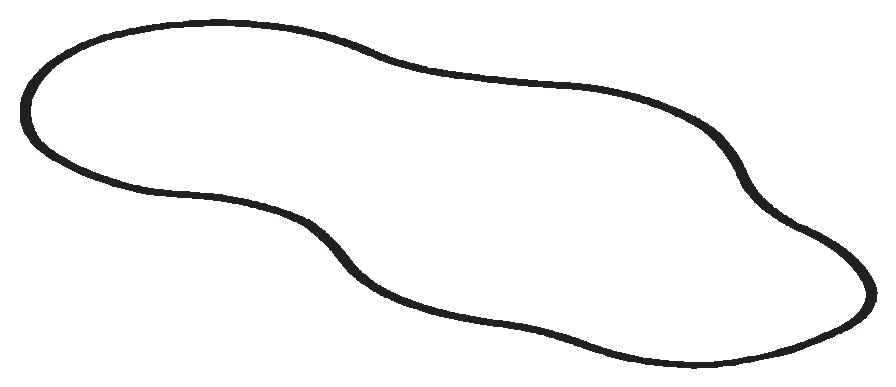
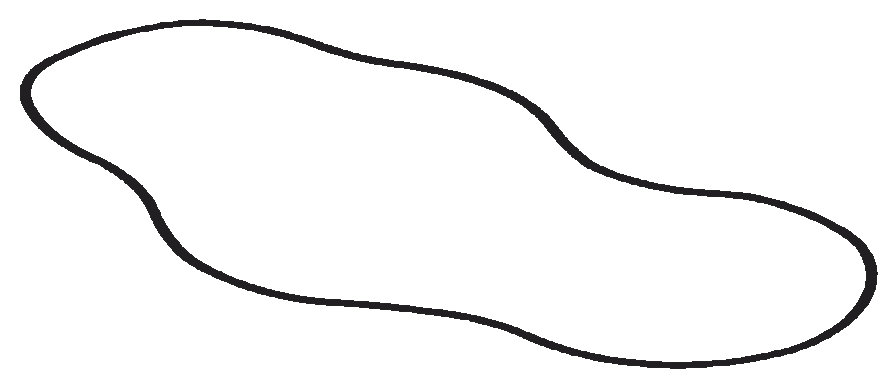
# SketchUp Ruby script. Lengths in inches.
U = 1.inch
M = Sketchup.active_model
def pt(a) = Geom::Point3d.new(a.map { |v| v * U })
def face(e, loops, mat)
  f = e.add_face(loops[0].map { |a| pt(a) })
  loops[1..].each { |l| e.add_face(l.map { |a| pt(a) }).erase! }
  f.material = f.back_material = mat if mat
  f
end
# faces: each face lists its corners as indices into pts; further lists are holes
def faces(e, pts, list, mat = nil) = list.each { |f| face(e, (f[0].is_a?(Array) ? f : [f]).map { |l| l.map { |i| pts[i] } }, mat) }
# xy, xz, yz: faces in a plane at the given z, y or x. An outline is a flat list of corners, or four numbers for a rectangle; further outlines are holes
def ring(l) = l.size == 4 ? [[l[0], l[1]], [l[2], l[1]], [l[2], l[3]], [l[0], l[3]]] : l.each_slice(2).to_a
def flat(e, list, mat, &to3) = list.each { |f| face(e, (f[0].is_a?(Array) ? f : [f]).map { |l| ring(l).map { |u, v| to3.(u, v) } }, mat) }
def xy(e, z, list, mat = nil) = flat(e, list, mat) { |x, y| [x, y, z] }
def xz(e, y, list, mat = nil) = flat(e, list, mat) { |x, z| [x, y, z] }
def yz(e, x, list, mat = nil) = flat(e, list, mat) { |y, z| [x, y, z] }
def lines(e, pts, list) = list.each { |a, b| e.add_line(pt(pts[a]), pt(pts[b])) }
# prism: a flat outline (further loops are holes) pulled along v
def prism(e, loops, v, mat = nil)
  f = face(e, loops, mat); d = Geom::Vector3d.new(v.map { |x| x * U })
  f.pushpull(f.normal.samedirection?(d) ? d.length : -d.length)
end
def box(e, o, s, mat = nil) = prism(e, [[o, [o[0] + s[0], o[1], o[2]], [o[0] + s[0], o[1] + s[1], o[2]], [o[0], o[1] + s[1], o[2]]]], [0, 0, s[2]], mat)
def at(x, y, z, deg = 0) = Geom::Transformation.translation(pt([x, y, z])) * Geom::Transformation.rotation(ORIGIN, Z_AXIS, deg.degrees)
def axes(o, x, y, z) = Geom::Transformation.new([*x, 0, *y, 0, *z, 0, *pt(o).to_a, 1])
def part(name) = M.definitions.add(name)
# library, detail: a bought-in or finely detailed component or shape, given as its bounding box
def library(name, o, s) = part(name).tap { |d| box(d.entities, o, s) }
def detail(e, o, s) = box(e.add_group.entities, o, s)
def put(e, d, t, mat = nil) = e.add_instance(d, t).tap { |i| i.material = mat if mat }
def group(e, t, mat = nil) = e.add_group.tap { |g| g.transformation = t; g.material = mat if mat }.entities
root = M.entities
M.materials.add("Marble_07_1K").color = [36, 34, 36]
xy(root,19,[[[347.23,772.58,347.79,772.58,348.02,772.59,348.13,772.6,348.24,772.6,348.79,772.65,348.99,772.67,349.09,772.69,349.18,772.7,349.28,772.71,349.36,772.72,349.45,772.74,349.61,772.76,349.6875,772.78,349.77,772.79,349.85,772.8,349.93,772.82,350,772.83,350.08,772.85,350.16,772.86,350.32,772.9,350.4,772.91,350.47,772.93,350.55,772.95,350.63,772.96,350.71,772.98,350.78,773,350.86,773.02,350.9375,773.04,351.02,773.06,351.09,773.08,351.33,773.14,351.4,773.16,351.56,773.2,351.63,773.23,351.79,773.27,351.86,773.29,351.9375,773.32,352.01,773.34,352.09,773.37,352.17,773.39,352.24,773.42,352.32,773.44,352.39,773.47,352.47,773.49,352.54,773.52,352.62,773.54,352.69,773.57,352.77,773.6,352.84,773.625,352.92,773.65,352.99,773.68,353.07,773.71,353.14,773.74,353.22,773.77,353.36,773.83,353.4375,773.86,353.51,773.89,353.65,773.95,353.73,773.98,353.8,774.01,353.875,774.04,353.95,774.08,354.11,774.14,354.19,774.18,354.35,774.24,354.4375,774.28,354.52,774.3125,354.61,774.35,354.69,774.38,354.78,774.41,354.86,774.44,354.95,774.47,355.03,774.51,355.12,774.54,355.2,774.5625,355.29,774.59,355.46,774.65,355.55,774.68,355.63,774.7,355.72,774.73,355.81,774.75,355.89,774.78,356.07,774.82,356.16,774.85,356.24,774.87,356.6,774.95,356.68,774.97,356.77,774.98,357.04,775.04,357.125,775.05,357.22,775.07,357.3,775.08,357.39,775.09,357.48,775.11,358.11,775.18,358.2,775.1875,358.29,775.2,358.38,775.2,358.47,775.21,358.5625,775.21,358.65,775.22,358.74,775.22,358.84,775.23,359.12,775.23,359.22,775.24,359.46,775.24,359.6,775.25,359.76,775.25,359.9375,775.26,360.14,775.27,360.36,775.29,360.6,775.31,360.85,775.33,361.39,775.39,361.67,775.43,361.96,775.48,362.24,775.53,362.52,775.59,362.8,775.66,363.08,775.74,363.35,775.82,363.625,775.91,363.9,776.01,364.17,776.11,364.4375,776.22,364.7,776.34,364.96,776.46,365.22,776.59,365.48,776.73,365.98,777.02,366.22,777.18,366.7,777.52,366.9375,777.7,367.17,777.9,367.41,778.11,367.64,778.35,367.875,778.6,368.11,778.875,368.35,779.18,368.59,779.52,368.85,779.9,369.11,780.34,369.4,780.85,369.7,781.4375,370.02,782.11,370.37,782.88,370.59,783.7,370.76,784.42,370.9,785.05,371.01,785.59,371.09,786.06,371.15,786.45,371.19,786.79,371.22,787.07,371.25,787.3,371.26,787.49,371.28,787.65,371.29,787.78,371.29,788.17,371.28,788.23,371.28,788.36,371.27,788.43,371.27,788.49,371.26,788.56,371.25,788.62,371.24,788.6875,371.24,788.75,371.23,788.81,371.22,788.88,371.21,788.94,371.2,789.01,371.18,789.07,371.17,789.13,371.16,789.2,371.14,789.26,371.13,789.32,371.12,789.39,371.08,789.51,371.07,789.58,371.01,789.76,370.99,789.83,370.89,790.13,370.86,790.19,370.84,790.25,370.8125,790.3125,370.79,790.375,370.76,790.43,370.74,790.49,370.65,790.67,370.625,790.73,370.51,790.96,370.47,791.01,370.44,791.07,370.41,791.125,370.375,791.18,370.34,791.24,370.31,791.29,370.27,791.35,370.24,791.4,370.2,791.46,370.16,791.51,370.125,791.5625,370.09,791.61,370.05,791.67,369.73,792.07,369.68,792.12,369.64,792.17,369.55,792.26,369.51,792.3125,369.46,792.36,369.41,792.4,369.37,792.45,369.32,792.49,369.23,792.58,369.13,792.67,369.03,792.75,368.99,792.79,368.9375,792.83,368.89,792.87,368.84,792.91,368.8,792.94,368.7,793.02,368.66,793.05,368.61,793.09,368.53,793.15,368.5,793.18,368.46,793.2,368.43,793.22,368.41,793.24,368.38,793.26,368.35,793.29,368.33,793.3,368.32,793.31,368.3,793.32,368.28,793.34,368.27,793.34,368.25,793.35,368.24,793.37,368.22,793.38,368.16,793.42,368.125,793.44,368.08,793.47,367.98,793.55,367.92,793.59,367.78,793.67,367.71,793.72,367.64,793.76,367.57,793.81,367.5,793.85,367.43,793.9,367.36,793.9375,367.28,793.98,367.21,794.03,367.07,794.11,366.99,794.15,366.85,794.23,366.77,794.27,366.7,794.31,366.62,794.35,366.55,794.39,366.47,794.43,366.4,794.46,366.32,794.5,366.25,794.54,366.17,794.57,366.09,794.61,366.02,794.64,365.94,794.68,365.86,794.71,365.79,794.74,365.71,794.78,365.55,794.84,365.48,794.875,365.4,794.9,364.84,795.11,364.76,795.13,364.68,795.16,364.6,795.1875,364.52,795.21,364.44,795.24,364.36,795.26,364.28,795.29,364.04,795.35,363.88,795.4,363.8,795.42,363.71,795.4375,363.63,795.46,363.39,795.52,363.3,795.53,363.14,795.57,363.06,795.58,362.97,795.6,362.89,795.61,362.81,795.63,362.73,795.64,362.64,795.66,362.48,795.68,362.39,795.69,362.3125,795.7,362.23,795.71,362.15,795.73,362.0625,795.73,361.98,795.74,361.9,795.75,361.81,795.76,361.65,795.78,361.56,795.78,361.47,795.79,361.17,795.82,360.95,795.84,360.83,795.85,360.71,795.87,360.47,795.89,359.99,795.97,359.76,796.01,359.64,796.03,359.52,796.06,359.4,796.08,359.28,796.11,359.17,796.14,359.05,796.16,358.93,796.19,358.82,796.23,358.7,796.26,358.59,796.29,358.47,796.33,358.36,796.36,358.24,796.4,358.13,796.4375,358.01,796.48,357.9,796.52,357.79,796.5625,357.68,796.6,357.5625,796.65,357.45,796.69,357.01,796.89,356.9,796.9375,356.79,796.99,356.68,797.04,356.58,797.1,356.47,797.15,356.36,797.21,356.26,797.27,356.15,797.32,356.05,797.38,355.94,797.44,355.84,797.51,355.64,797.63,355.53,797.7,355.43,797.76,355.13,797.97,355.04,798.04,354.9375,798.11,354.84,798.18,354.74,798.25,354.65,798.33,354.55,798.4,354.46,798.47,354.29,798.61,354.02,798.82,353.93,798.9,353.71,799.08,353.57,799.19,353.42,799.3,353.27,799.42,353.14,799.52,353.02,799.61,352.91,799.6875,352.81,799.75,352.73,799.8125,352.65,799.87,352.51,799.97,352.45,800.01,352.38,800.05,352.32,800.1,352.26,800.14,352.21,800.18,352.15,800.21,352.09,800.25,352.04,800.29,351.98,800.33,351.92,800.36,351.86,800.4,351.81,800.4375,351.75,800.47,351.69,800.51,351.63,800.54,351.58,800.58,351.52,800.62,351.46,800.65,351.4,800.6875,351.34,800.72,351.29,800.76,351.23,800.79,351.17,800.83,351.11,800.86,351.05,800.9,350.93,800.96,350.875,801,350.82,801.03,350.76,801.06,350.7,801.1,350.58,801.16,350.52,801.2,350.46,801.23,350.41,801.26,350.35,801.29,350.3,801.3125,350.25,801.34,350.21,801.36,350.16,801.39,350.08,801.43,350.05,801.45,350.01,801.46,349.97,801.48,349.94,801.5,349.91,801.51,349.83,801.55,349.8,801.56,349.76,801.58,349.73,801.6,349.69,801.61,349.66,801.63,349.62,801.64,349.59,801.66,349.55,801.68,349.51,801.69,349.47,801.71,349.43,801.72,349.35,801.76,349.2,801.82,349.13,801.84,349.0625,801.87,348.98,801.9,348.89,801.93,348.79,801.97,348.68,802,348.59,802.03,348.51,802.05,348.4375,802.07,348.375,802.09,348.32,802.11,348.26,802.12,348.22,802.13,348.17,802.14,348.125,802.16,348.08,802.17,348,802.19,347.97,802.19,347.85,802.22,347.8125,802.23,347.78,802.24,347.74,802.24,347.62,802.27,347.58,802.27,347.55,802.28,347.47,802.3,347.43,802.3,347.39,802.31,347.35,802.3125,347.28,802.33,347.24,802.33,347.2,802.34,347.16,802.34,347.125,802.35,347.09,802.35,347.05,802.36,347.01,802.36,346.97,802.37,346.89,802.38,346.85,802.38,346.8,802.39,346.74,802.39,346.67,802.4,346.59,802.41,346.49,802.42,346.38,802.43,346.25,802.4375,346.1,802.45,345.9375,802.46,345.76,802.47,345.56,802.48,345.34,802.49,345.11,802.5,344.85,802.51,344.58,802.52,344.29,802.52,343.99,802.51,343.67,802.5,343.34,802.47,342.99,802.4375,342.63,802.39,342.3,802.32,342.01,802.26,341.76,802.2,341.55,802.15,341.36,802.11,341.21,802.07,341.07,802.03,340.96,802,340.87,801.97,340.79,801.95,340.72,801.93,340.66,801.92,340.61,801.9,340.57,801.89,340.54,801.88,340.5,801.87,340.47,801.86,340.44,801.84,340.4,801.83,340.37,801.82,340.33,801.81,340.27,801.79,340.23,801.77,340.17,801.75,340.13,801.74,340.1,801.73,340.07,801.71,340.03,801.7,339.97,801.68,339.94,801.66,339.9,801.65,339.87,801.64,339.84,801.625,339.8,801.61,339.74,801.59,339.71,801.57,339.67,801.56,339.64,801.54,339.61,801.53,339.57,801.52,339.54,801.5,339.48,801.48,339.44,801.46,339.41,801.45,339.38,801.43,339.35,801.42,339.3125,801.4,339.28,801.39,339.24,801.37,339.21,801.35,339.17,801.33,339.125,801.3125,339.08,801.29,339.03,801.27,338.98,801.24,338.92,801.21,338.85,801.17,338.77,801.13,338.68,801.09,338.59,801.04,338.45,800.96,338.39,800.92,338.34,800.89,338.29,800.87,338.25,800.84,338.17,800.8,338.14,800.77,338.11,800.75,338.07,800.73,338.04,800.71,338.01,800.7,337.95,800.66,337.93,800.64,337.89,800.62,337.86,800.6,337.78,800.54,337.72,800.51,337.65,800.47,337.57,800.42,337.48,800.37,337.375,800.3,337.26,800.23,337.13,800.16,337,800.08,336.86,800,336.71,799.91,336.57,799.83,336.42,799.75,336.27,799.66,335.97,799.5,335.83,799.42,335.53,799.26,335.375,799.18,335.23,799.1,335.08,799.02,334.92,798.95,334.77,798.87,334.62,798.8,334.47,798.72,334.31,798.65,334.16,798.57,334.01,798.5,333.85,798.43,333.55,798.29,333.41,798.22,333.27,798.16,333.14,798.1,333.02,798.04,332.91,797.99,332.81,797.94,332.71,797.9,332.625,797.85,332.54,797.8125,332.46,797.77,332.38,797.74,332.31,797.7,332.23,797.67,332.15,797.63,332.08,797.6,332,797.57,331.93,797.54,331.85,797.5,331.78,797.47,331.62,797.41,331.55,797.38,331.39,797.32,331.32,797.29,331.24,797.27,331.08,797.21,331.01,797.1875,330.93,797.16,330.85,797.13,330.77,797.11,330.69,797.08,330.62,797.06,330.54,797.04,330.46,797.01,330.14,796.93,330.0625,796.91,329.98,796.89,329.5,796.77,329.41,796.76,329.23,796.72,329.13,796.7,329.02,796.68,328.91,796.67,328.79,796.65,328.65,796.625,328.49,796.6,328.3125,796.58,328.11,796.56,327.88,796.53,327.65,796.52,327.45,796.51,327.27,796.5,327.11,796.5,326.97,796.49,326.62,796.49,326.52,796.5,326.25,796.5,326.16,796.51,326.07,796.51,325.99,796.52,325.9,796.52,325.82,796.53,325.73,796.53,325.64,796.54,325.54,796.55,325.4375,796.55,325.33,796.56,324.78,796.56,324.62,796.55,324.45,796.55,324.28,796.54,324.1,796.53,323.92,796.51,323.73,796.5,323.37,796.46,323.18,796.4375,323,796.41,322.82,796.39,322.64,796.36,322.46,796.32,322.28,796.29,321.74,796.17,321.5625,796.125,321.39,796.08,321.03,795.98,320.86,795.93,320.68,795.87,320.51,795.8125,320.34,795.75,320.16,795.69,319.82,795.56,319.48,795.42,319.32,795.34,319.15,795.27,318.98,795.1875,318.82,795.11,318.65,795.03,317.85,794.58,317.7,794.48,317.54,794.39,317.39,794.29,317.23,794.1875,317.08,794.08,316.93,793.98,316.78,793.87,316.64,793.76,316.49,793.65,316.35,793.54,316.2,793.42,316.0625,793.3,315.92,793.19,315.79,793.0625,315.65,792.94,315.51,792.82,315.38,792.69,315.25,792.5625,315.12,792.43,314.99,792.3,314.87,792.17,314.74,792.04,314.26,791.48,314.15,791.34,314.03,791.19,313.92,791.05,313.8125,790.9,313.7,790.75,313.6,790.6,313.49,790.45,313.39,790.29,313.28,790.13,313.17,789.96,313.0625,789.78,312.95,789.59,312.83,789.39,312.72,789.19,312.48,788.77,312.26,788.35,312.16,788.14,312.07,787.94,311.99,787.75,311.92,787.57,311.86,787.39,311.8,787.22,311.75,787.05,311.63,786.57,311.6,786.41,311.56,786.25,311.54,786.09,311.51,785.9375,311.48,785.78,311.42,785.3,311.41,785.15,311.39,784.99,311.38,784.84,311.37,784.6875,311.36,784.54,311.36,784.4,311.35,784.27,311.35,783.81,311.36,783.71,311.36,783.53,311.37,783.45,311.37,783.36,311.38,783.28,311.38,783.2,311.39,783.12,311.39,783.03,311.4,782.9375,311.41,782.84,311.42,782.74,311.4375,782.625,311.46,782.5,311.48,782.37,311.52,782.09,311.55,781.9375,311.58,781.79,311.61,781.63,311.65,781.47,311.68,781.32,311.72,781.16,311.76,781.01,311.81,780.85,311.85,780.7,311.9,780.55,311.95,780.39,312.05,780.09,312.29,779.49,312.35,779.35,312.49,779.05,312.63,778.77,312.7,778.62,312.78,778.47,312.96,778.17,313.06,778.01,313.16,777.84,313.27,777.67,313.4,777.48,313.54,777.28,313.7,777.0625,313.89,776.82,314.11,776.54,314.36,776.24,314.66,775.89,314.99,775.59,315.3,775.33,315.57,775.1,315.81,774.9,316.03,774.74,316.24,774.59,316.43,774.46,316.61,774.34,316.78,774.24,316.96,774.14,317.13,774.04,317.32,773.96,317.51,773.87,317.71,773.79,317.92,773.71,318.16,773.63,318.41,773.55,318.68,773.47,318.97,773.4,319.28,773.32,319.59,773.25,319.91,773.1875,320.24,773.13,320.58,773.08,320.91,773.04,321.25,773,321.58,772.98,321.92,772.96,322.59,772.96,322.93,772.97,323.27,772.99,323.93,773.05,324.26,773.09,324.57,773.14,324.87,773.1875,325.15,773.24,325.42,773.29,325.65,773.35,325.87,773.4,326.23,773.5,326.39,773.55,326.54,773.61,326.68,773.67,326.83,773.74,326.99,773.8125,327.15,773.9,327.32,773.99,327.5,774.08,327.68,774.18,327.87,774.28,328.05,774.39,328.24,774.49,328.42,774.6,328.6,774.7,328.77,774.8,328.9375,774.89,329.1,774.99,329.27,775.08,329.43,775.17,329.59,775.25,329.75,775.34,329.92,775.42,330.08,775.49,330.24,775.57,330.4,775.64,330.74,775.78,330.9,775.84,331.07,775.91,331.24,775.97,331.41,776.02,331.58,776.08,332.09,776.23,332.26,776.27,332.4375,776.32,332.61,776.36,332.79,776.39,332.96,776.43,333.14,776.46,333.3125,776.49,333.49,776.52,333.67,776.54,333.84,776.5625,334.02,776.58,334.2,776.6,334.55,776.62,334.73,776.63,334.91,776.63,335.09,776.64,335.4375,776.64,335.61,776.63,335.78,776.625,335.9375,776.62,336.09,776.61,336.23,776.6,336.36,776.58,336.48,776.57,336.58,776.56,336.66,776.54,336.74,776.53,336.8,776.52,336.86,776.5,336.91,776.48,336.96,776.47,337.06,776.43,337.1,776.42,337.15,776.4,337.21,776.38,337.56,776.24,337.62,776.22,337.97,776.08,338.03,776.06,338.13,776.02,338.18,775.99,338.38,775.91,338.4375,775.88,338.49,775.86,338.55,775.83,338.61,775.81,338.73,775.75,338.8,775.72,338.96,775.64,339.06,775.6,339.17,775.55,339.69,775.29,339.8,775.23,339.89,775.18,339.98,775.14,340.12,775.06,340.18,775.03,340.24,774.99,340.3,774.96,340.4,774.9,340.5,774.85,340.65,774.76,340.7,774.74,340.74,774.71,340.84,774.65,340.89,774.625,340.93,774.6,341.18,774.45,341.24,774.41,341.36,774.34,341.43,774.3,341.51,774.25,341.59,774.21,341.67,774.16,341.76,774.11,341.86,774.06,341.95,774,342.75,773.6,342.86,773.56,342.96,773.51,343.0625,773.47,343.17,773.43,343.27,773.38,343.48,773.3,343.59,773.26,343.69,773.23,343.91,773.15,344.02,773.12,344.12,773.09,344.23,773.05,344.67,772.93,344.77,772.91,344.88,772.88,344.99,772.86,345.1,772.83,345.21,772.81,345.33,772.79,345.4375,772.77,345.55,772.75,345.88,772.69,346.1,772.67,346.22,772.65,346.55,772.62,346.67,772.61,346.78,772.6,346.89,772.6,347,772.59,347.12,772.59],[347.35,773.18,347.24,773.1875,347.14,773.19,347.03,773.19,346.92,773.2,346.82,773.21,346.71,773.21,346.6,773.22,346.5,773.23,346.28,773.25,346.18,773.26,346.07,773.28,345.97,773.29,345.86,773.31,345.75,773.32,345.65,773.34,345.54,773.36,345.4375,773.38,345.33,773.4,345.23,773.42,345.125,773.45,345.02,773.47,344.92,773.49,344.8125,773.52,344.71,773.55,344.61,773.57,344.5,773.6,344.3,773.66,344.2,773.7,344.1,773.73,343.99,773.76,343.89,773.8,343.79,773.83,343.39,773.99,343.3,774.03,343,774.15,342.9,774.2,342.81,774.24,342.71,774.29,342.62,774.34,342.52,774.38,342.43,774.43,342.33,774.48,341.97,774.68,341.89,774.73,341.8125,774.78,341.74,774.82,341.67,774.86,341.61,774.9,341.49,774.96,341.44,775,341.24,775.12,341.19,775.14,341.15,775.17,340.9,775.32,340.85,775.34,340.65,775.46,340.6,775.48,340.45,775.57,340.41,775.59,340.31,775.65,340.26,775.67,340.16,775.73,340.1,775.75,340.05,775.78,340,775.8,339.9,775.86,339.85,775.88,339.8,775.91,339.75,775.93,339.7,775.96,339.65,775.98,339.6,776.01,339.55,776.03,339.5,776.06,339.45,776.08,339.4,776.11,339.34,776.13,339.29,776.16,339.19,776.2,339.14,776.23,339.09,776.25,339.04,776.28,338.98,776.3,338.93,776.32,338.88,776.35,338.78,776.39,338.73,776.42,338.67,776.4375,338.62,776.46,338.57,776.48,338.52,776.51,338.47,776.53,338.41,776.55,338.31,776.59,338.26,776.62,338.2,776.64,338.05,776.7,337.99,776.72,337.89,776.76,337.84,776.79,337.78,776.81,337.68,776.85,337.57,776.89,337.47,776.93,337.41,776.95,337.31,776.99,337.25,777.01,337.2,777.02,337.15,777.04,337.09,777.0625,337.03,777.08,336.89,777.12,336.8,777.13,336.71,777.15,336.59,777.17,336.46,777.18,336.32,777.19,336.17,777.21,336,777.22,335.82,777.23,335.64,777.23,335.46,777.24,334.9,777.24,334.52,777.22,334.34,777.21,334.15,777.2,333.96,777.18,333.78,777.16,333.59,777.14,333.4,777.11,333.22,777.08,333.03,777.05,332.85,777.02,332.66,776.98,332.48,776.95,332.3,776.9,332.12,776.86,331.93,776.8125,331.75,776.76,331.57,776.71,331.39,776.65,331.22,776.6,331.04,776.54,330.86,776.47,330.6875,776.41,330.51,776.34,330.17,776.2,329.99,776.12,329.65,775.96,329.49,775.88,329.15,775.7,328.99,775.61,328.65,775.43,328.31,775.23,327.95,775.03,327.77,774.92,327.23,774.62,326.89,774.44,326.74,774.36,326.59,774.29,326.45,774.23,326.32,774.17,326.18,774.12,326.03,774.07,325.87,774.02,325.69,773.98,325.5,773.93,325.27,773.88,325.02,773.83,324.76,773.78,324.47,773.73,324.17,773.6875,323.86,773.65,323.55,773.62,323.23,773.59,322.91,773.57,322.58,773.56,322.26,773.56,321.62,773.58,321.3,773.6,320.34,773.72,319.72,773.84,319.42,773.91,319.13,773.98,318.86,774.05,318.6,774.125,318.36,774.2,318.14,774.27,317.94,774.35,317.76,774.42,317.59,774.49,317.43,774.57,317.28,774.64,317,774.8,316.74,774.96,316.61,775.05,316.49,775.14,316.36,775.23,316.12,775.41,316,775.51,315.89,775.61,315.77,775.71,315.65,775.8125,315.54,775.92,315.42,776.03,315.29,776.15,315.17,776.28,315.04,776.41,314.91,776.55,314.76,776.71,314.61,776.88,314.45,777.08,314.26,777.3125,314.0625,777.58,313.84,777.88,313.59,778.23,313.39,778.61,313.07,779.25,312.95,779.51,312.84,779.75,312.75,779.96,312.68,780.16,312.61,780.35,312.55,780.52,312.49,780.6875,312.4375,780.85,312.39,781.01,312.35,781.16,312.31,781.3125,312.27,781.46,312.24,781.61,312.2,781.76,312.17,781.91,312.14,782.05,312.12,782.2,312.09,782.35,312.07,782.51,312.03,782.81,312.02,782.96,312,783.11,311.98,783.41,311.97,783.5625,311.97,783.72,311.96,783.87,311.96,784.32,311.97,784.48,311.97,784.63,311.99,784.93,312.01,785.08,312.02,785.23,312.04,785.39,312.06,785.54,312.08,785.6875,312.1,785.84,312.16,786.14,312.1875,786.29,312.22,786.43,312.25,786.58,312.33,786.88,312.375,787.04,312.43,787.2,312.49,787.36,312.55,787.53,312.63,787.71,312.72,787.9,312.8125,788.1,312.92,788.3,313.02,788.5,313.13,788.7,313.25,788.9,313.36,789.1,313.58,789.46,313.68,789.64,313.79,789.8,313.89,789.96,314.09,790.26,314.19,790.4,314.3,790.54,314.4,790.68,314.73,791.1,314.84,791.23,314.95,791.37,315.07,791.5,315.1875,791.63,315.31,791.76,315.43,791.88,315.55,792.01,315.8,792.26,315.93,792.375,316.05,792.5,316.19,792.61,316.32,792.73,316.45,792.84,316.59,792.95,316.72,793.0625,316.86,793.17,317,793.28,317.14,793.38,317.28,793.49,317.43,793.59,317.57,793.6875,317.72,793.78,317.86,793.88,318.01,793.97,318.16,794.0625,318.3125,794.15,318.47,794.24,318.62,794.32,318.77,794.41,319.09,794.57,319.24,794.64,319.4,794.72,319.5625,794.79,319.72,794.86,319.88,794.93,320.05,795,320.21,795.0625,320.375,795.125,320.54,795.18,320.7,795.24,320.87,795.3,321.21,795.4,321.54,795.5,321.88,795.58,322.05,795.625,322.23,795.66,322.4,795.7,322.74,795.76,322.92,795.79,323.09,795.82,323.26,795.84,323.4375,795.86,323.61,795.88,323.79,795.9,324.13,795.92,324.3,795.94,324.47,795.94,324.63,795.95,324.79,795.95,324.93,795.96,325.07,795.96,325.19,795.95,325.42,795.95,325.52,795.94,325.61,795.9375,325.7,795.93,325.79,795.92,325.87,795.92,325.96,795.91,326.04,795.91,326.13,795.9,326.3,795.9,326.39,795.89,327.16,795.89,327.24,795.9,327.42,795.9,327.5,795.91,327.59,795.91,327.67,795.92,327.76,795.92,327.84,795.93,327.93,795.9375,328.02,795.94,328.1,795.95,328.1875,795.96,328.27,795.97,328.36,795.98,328.44,795.99,328.53,796,328.61,796.01,328.7,796.02,328.78,796.03,328.87,796.05,328.95,796.06,329.04,796.07,329.12,796.09,329.21,796.1,329.29,796.12,329.375,796.13,329.46,796.15,329.54,796.17,329.63,796.18,329.71,796.2,329.8,796.22,329.96,796.26,330.05,796.28,330.21,796.32,330.3,796.34,330.38,796.36,330.46,796.39,330.54,796.41,330.625,796.43,330.71,796.46,330.79,796.48,330.875,796.51,330.95,796.53,331.04,796.56,331.12,796.59,331.2,796.61,331.44,796.7,331.53,796.73,331.61,796.76,331.7,796.79,331.88,796.87,331.98,796.9,332.08,796.95,332.1875,796.99,332.31,797.04,332.44,797.1,332.59,797.17,332.76,797.25,332.96,797.34,333.17,797.45,333.61,797.65,334,797.83,334.34,797.99,334.64,798.14,334.91,798.27,335.14,798.38,335.36,798.49,335.74,798.69,335.92,798.78,336.09,798.875,336.25,798.96,336.41,799.05,336.5625,799.13,336.71,799.22,336.86,799.3,337.16,799.48,337.44,799.64,337.57,799.72,337.6875,799.79,337.8,799.85,337.89,799.91,337.97,799.96,338.04,800,338.1,800.03,338.14,800.0625,338.18,800.09,338.22,800.11,338.31,800.17,338.33,800.18,338.42,800.24,338.45,800.25,338.48,800.27,338.5,800.29,338.53,800.31,338.5625,800.32,338.59,800.34,338.62,800.36,338.68,800.39,338.71,800.41,338.73,800.43,338.76,800.44,338.82,800.48,338.85,800.49,338.89,800.51,338.95,800.55,339.11,800.63,339.16,800.66,339.22,800.6875,339.29,800.72,339.36,800.76,339.45,800.8,339.53,800.84,339.61,800.87,339.73,800.93,339.79,800.95,339.83,800.97,339.92,801.01,339.95,801.02,339.99,801.04,340.02,801.05,340.06,801.0625,340.09,801.08,340.18,801.11,340.22,801.125,340.25,801.14,340.4,801.19,340.44,801.21,340.53,801.24,340.5625,801.25,340.59,801.26,340.66,801.28,340.6875,801.29,340.72,801.3,340.75,801.3125,340.79,801.32,340.83,801.34,340.92,801.36,340.98,801.38,341.05,801.4,341.125,801.42,341.21,801.44,341.3,801.47,341.4,801.49,341.51,801.52,341.61,801.55,341.72,801.57,341.84,801.6,341.95,801.63,342.0625,801.65,342.17,801.68,342.29,801.7,342.4,801.72,342.51,801.75,342.74,801.79,342.85,801.81,342.97,801.83,343.09,801.84,343.21,801.86,343.47,801.89,343.61,801.9,343.77,801.91,343.93,801.91,344.1,801.92,344.66,801.92,344.85,801.91,345.04,801.91,345.23,801.9,345.59,801.88,345.91,801.86,346.0625,801.85,346.2,801.84,346.86,801.77,346.93,801.77,346.97,801.76,347.01,801.76,347.04,801.75,347.08,801.75,347.11,801.74,347.15,801.74,347.1875,801.73,347.22,801.72,347.26,801.72,347.29,801.71,347.33,801.71,347.37,801.7,347.4,801.69,347.4375,801.6875,347.47,801.68,347.51,801.67,347.54,801.67,347.62,801.65,347.65,801.65,347.6875,801.64,347.72,801.63,347.76,801.62,347.79,801.61,347.83,801.61,347.86,801.6,347.94,801.58,347.97,801.57,348.01,801.5625,348.04,801.55,348.08,801.55,348.11,801.54,348.15,801.53,348.18,801.52,348.22,801.51,348.25,801.5,348.29,801.49,348.32,801.48,348.36,801.47,348.39,801.46,348.43,801.45,348.46,801.44,348.5,801.42,348.56,801.4,348.6,801.39,348.63,801.38,348.67,801.37,348.7,801.36,348.74,801.34,348.77,801.33,348.81,801.32,348.84,801.31,348.875,801.3,348.91,801.28,348.94,801.27,348.98,801.26,349.01,801.24,349.04,801.23,349.08,801.22,349.11,801.2,349.15,801.19,349.18,801.18,349.21,801.16,349.25,801.15,349.28,801.14,349.3125,801.12,349.35,801.11,349.38,801.09,349.41,801.08,349.45,801.0625,349.48,801.05,349.51,801.03,349.55,801.02,349.58,801,349.61,800.99,349.64,800.97,349.68,800.95,349.71,800.9375,349.74,800.92,349.78,800.91,349.8125,800.89,349.85,800.87,349.93,800.83,349.97,800.8,350.02,800.78,350.07,800.75,350.12,800.73,350.17,800.7,350.23,800.67,350.29,800.63,350.34,800.6,350.52,800.51,350.58,800.47,350.63,800.44,350.69,800.41,350.75,800.375,350.8,800.34,350.86,800.31,350.92,800.27,350.98,800.24,351.03,800.21,351.09,800.17,351.15,800.14,351.2,800.1,351.26,800.07,351.31,800.03,351.37,800,351.43,799.96,351.48,799.93,351.54,799.89,351.59,799.85,351.65,799.82,351.71,799.78,351.76,799.75,351.82,799.71,351.87,799.67,351.93,799.64,351.98,799.6,352.04,799.5625,352.09,799.52,352.15,799.49,352.25,799.41,352.31,799.375,352.36,799.34,352.42,799.3,352.52,799.22,352.58,799.18,352.68,799.1,352.74,799.0625,352.79,799.02,352.84,798.98,352.9,798.94,353,798.86,353.06,798.82,353.26,798.66,353.32,798.62,353.47,798.5,353.52,798.45,353.57,798.41,353.63,798.37,353.68,798.32,353.74,798.27,353.81,798.22,353.87,798.17,353.94,798.11,354.02,798.05,354.38,797.77,354.48,797.69,354.58,797.62,354.69,797.55,354.79,797.47,354.89,797.4,355,797.33,355.1,797.26,355.21,797.19,355.3125,797.12,355.42,797.05,355.53,796.99,355.64,796.92,356.3,796.56,356.42,796.5,356.53,796.45,356.64,796.39,356.76,796.34,356.875,796.29,356.99,796.23,357.11,796.18,357.22,796.14,357.46,796.04,357.58,796,357.69,795.95,357.8125,795.91,357.93,795.87,358.41,795.71,358.54,795.68,358.66,795.64,359.02,795.55,359.15,795.52,359.27,795.49,359.39,795.47,359.52,795.44,359.64,795.42,359.77,795.39,359.89,795.37,360.02,795.35,360.14,795.33,360.27,795.3125,360.39,795.3,360.52,795.28,360.64,795.27,360.76,795.25,360.88,795.24,360.99,795.23,361.11,795.22,361.21,795.21,361.3125,795.2,361.41,795.19,361.5,795.18,361.58,795.18,361.67,795.17,361.91,795.14,361.99,795.14,362.07,795.125,362.15,795.12,362.31,795.1,362.39,795.08,362.63,795.05,362.71,795.03,362.79,795.02,362.86,795,362.94,794.99,363.02,794.97,363.1,794.96,363.18,794.94,363.26,794.93,363.34,794.91,363.41,794.89,363.65,794.83,363.73,794.8125,363.8,794.79,364.04,794.73,364.11,794.71,364.19,794.68,364.27,794.66,364.34,794.64,364.42,794.61,364.5,794.59,364.57,794.5625,364.65,794.54,364.72,794.51,364.8,794.48,364.875,794.46,364.95,794.43,365.03,794.4,365.1,794.37,365.18,794.34,365.25,794.3125,365.33,794.28,365.47,794.22,365.55,794.19,365.62,794.16,365.69,794.125,365.77,794.09,365.91,794.03,365.99,793.99,366.06,793.96,366.13,793.92,366.2,793.89,366.27,793.85,366.35,793.8125,366.42,793.78,367.05,793.42,367.11,793.38,367.25,793.3,367.32,793.25,367.39,793.21,367.45,793.17,367.52,793.125,367.58,793.08,367.64,793.05,367.69,793.01,367.74,792.98,367.78,792.95,367.87,792.89,367.89,792.875,367.9,792.86,367.92,792.86,367.93,792.85,367.9375,792.84,367.95,792.83,367.96,792.82,367.98,792.8125,367.99,792.8,368.01,792.79,368.03,792.77,368.05,792.76,368.07,792.74,368.1,792.72,368.13,792.69,368.17,792.67,368.29,792.58,368.33,792.54,368.375,792.51,368.42,792.47,368.46,792.4375,368.55,792.37,368.6,792.33,368.64,792.29,368.6875,792.25,368.73,792.21,368.78,792.18,368.86,792.1,368.91,792.06,368.95,792.02,368.99,791.97,369.15,791.81,369.19,791.76,369.23,791.72,369.27,791.67,369.35,791.59,369.38,791.54,369.42,791.49,369.46,791.45,369.49,791.4,369.53,791.36,369.57,791.31,369.63,791.21,369.67,791.17,369.73,791.07,369.77,791.02,369.98,790.67,370.01,790.61,370.03,790.5625,370.06,790.51,370.09,790.46,370.11,790.41,370.14,790.35,370.16,790.3,370.1875,790.25,370.21,790.19,370.23,790.14,370.26,790.08,370.28,790.03,370.3,789.97,370.32,789.92,370.34,789.86,370.36,789.81,370.38,789.75,370.4,789.7,370.42,789.64,370.44,789.59,370.45,789.53,370.47,789.47,370.48,789.42,370.5,789.36,370.51,789.3,370.53,789.25,370.54,789.1875,370.56,789.13,370.57,789.07,370.58,789.02,370.61,788.84,370.62,788.79,370.65,788.61,370.65,788.55,370.66,788.49,370.66,788.4375,370.67,788.38,370.67,788.32,370.68,788.26,370.68,788.14,370.6875,788.08,370.6875,787.89,370.69,787.8125,370.68,787.72,370.67,787.6,370.66,787.47,370.64,787.31,370.625,787.12,370.6,786.91,370.57,786.68,370.54,786.43,370.46,785.89,370.36,785.33,370.3,785.04,370.23,784.76,370.17,784.48,370.09,784.2,370.01,783.93,369.93,783.65,369.75,783.1,369.65,782.83,369.54,782.5625,369.43,782.3,369.32,782.03,369.08,781.51,368.82,780.99,368.68,780.74,368.53,780.49,368.39,780.24,368.23,780,367.91,779.54,367.55,779.1,367.17,778.7,366.97,778.51,366.76,778.33,366.55,778.16,366.33,777.99,366.11,777.83,365.65,777.53,365.42,777.39,365.18,777.26,364.94,777.125,364.7,777,364.45,776.89,364.2,776.77,363.95,776.67,363.69,776.57,363.43,776.48,363.16,776.39,362.89,776.32,362.6,776.24,362.3,776.18,361.99,776.11,361.66,776.06,361.31,776.01,360.96,775.97,360.59,775.93,359.87,775.87,359.53,775.85,359.2,775.84,358.9,775.84,358.64,775.82,358.4,775.81,358.2,775.79,358.02,775.78,357.86,775.76,357.71,775.74,357.58,775.73,357.46,775.71,357.35,775.7,357.13,775.66,357.03,775.65,356.94,775.63,356.84,775.61,356.75,775.59,356.65,775.58,356.47,775.54,356.28,775.5,356.19,775.48,356.1,775.45,355.92,775.41,355.82,775.38,355.73,775.36,355.64,775.33,355.55,775.31,355.28,775.22,355.19,775.2,354.92,775.11,354.83,775.07,354.65,775.01,354.57,774.98,354.48,774.94,354.39,774.91,354.21,774.84,354.13,774.8,354.04,774.77,353.96,774.73,353.8,774.67,353.72,774.63,353.64,774.6,353.5,774.54,353.42,774.51,353.07,774.36,352.99,774.33,352.85,774.27,352.78,774.25,352.71,774.22,352.63,774.19,352.5625,774.17,352.49,774.14,352.42,774.11,352.34,774.09,352.27,774.0625,352.2,774.04,352.125,774.01,352.05,773.99,351.98,773.96,351.91,773.94,351.83,773.92,351.76,773.89,351.68,773.87,351.54,773.83,351.46,773.81,351.39,773.78,351.32,773.76,351.24,773.74,351.17,773.72,351.09,773.7,351.02,773.68,350.94,773.66,350.87,773.64,350.79,773.625,350.72,773.61,350.64,773.59,350.57,773.57,350.49,773.55,350.42,773.54,350.34,773.52,350.27,773.5,350.19,773.49,350.12,773.47,350.04,773.46,349.97,773.44,349.89,773.43,349.81,773.41,349.74,773.4,349.66,773.38,349.59,773.37,349.51,773.36,349.43,773.34,349.19,773.31,349.1,773.3,349.01,773.28,348.83,773.26,348.73,773.25,348.52,773.23,348.42,773.22,348.31,773.21,348.2,773.21,348.1,773.2,347.99,773.19,347.88,773.19,347.67,773.18]]],"Marble_07_1K")
